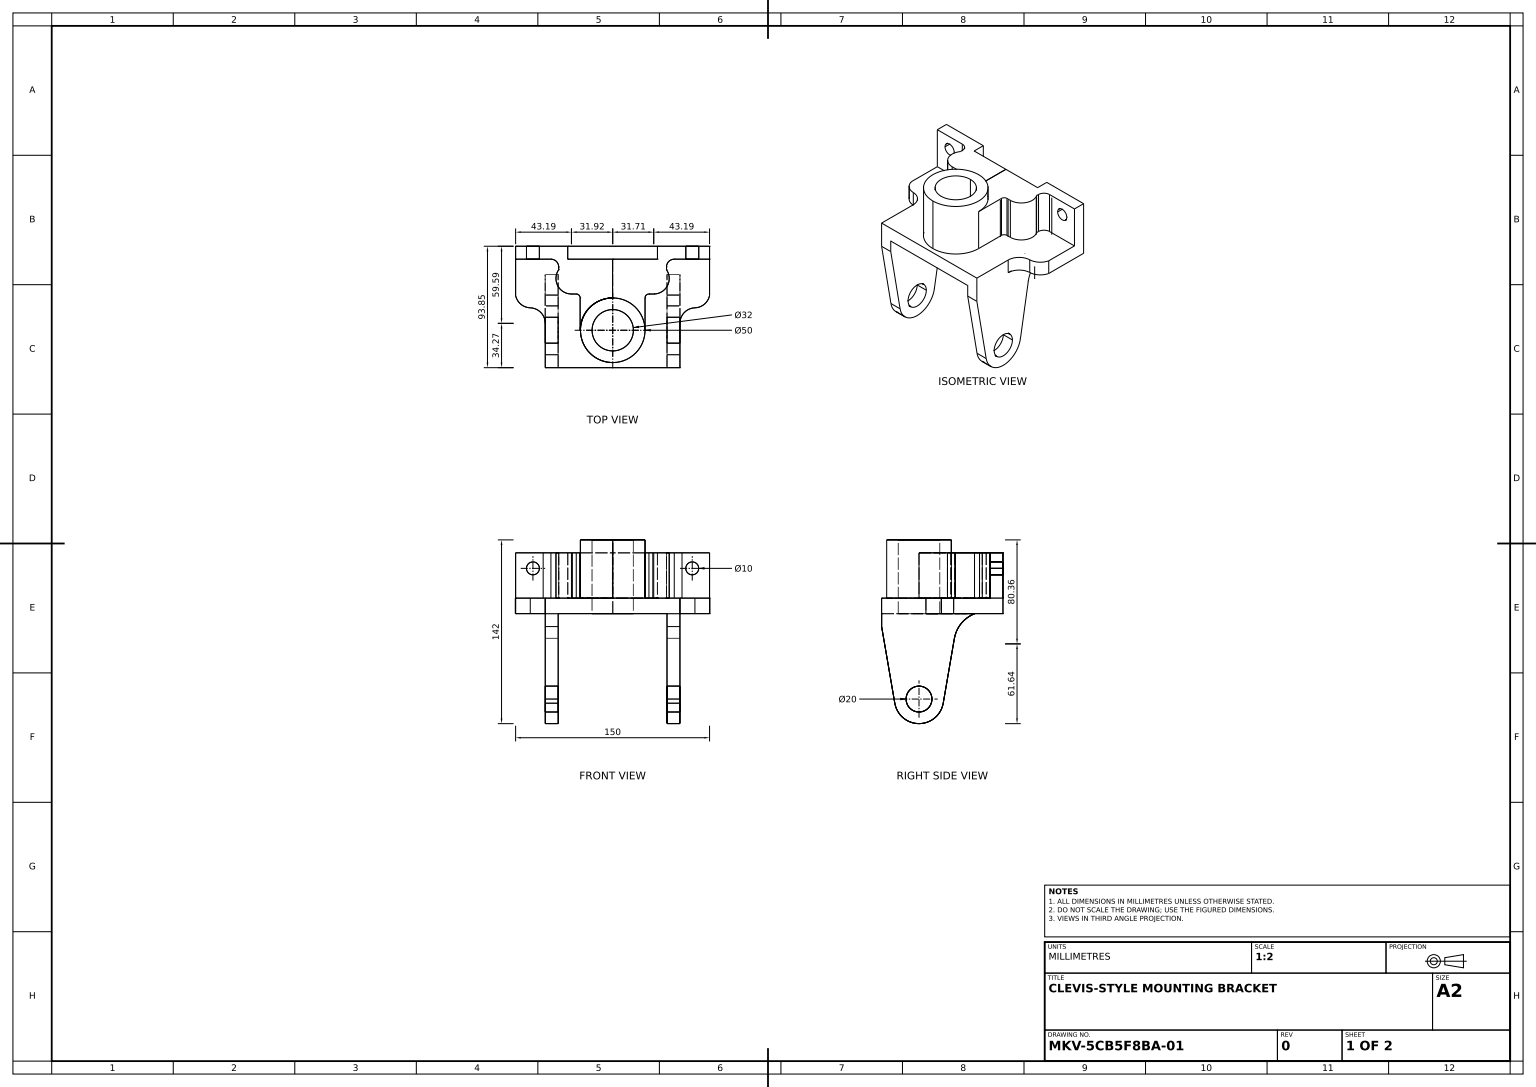
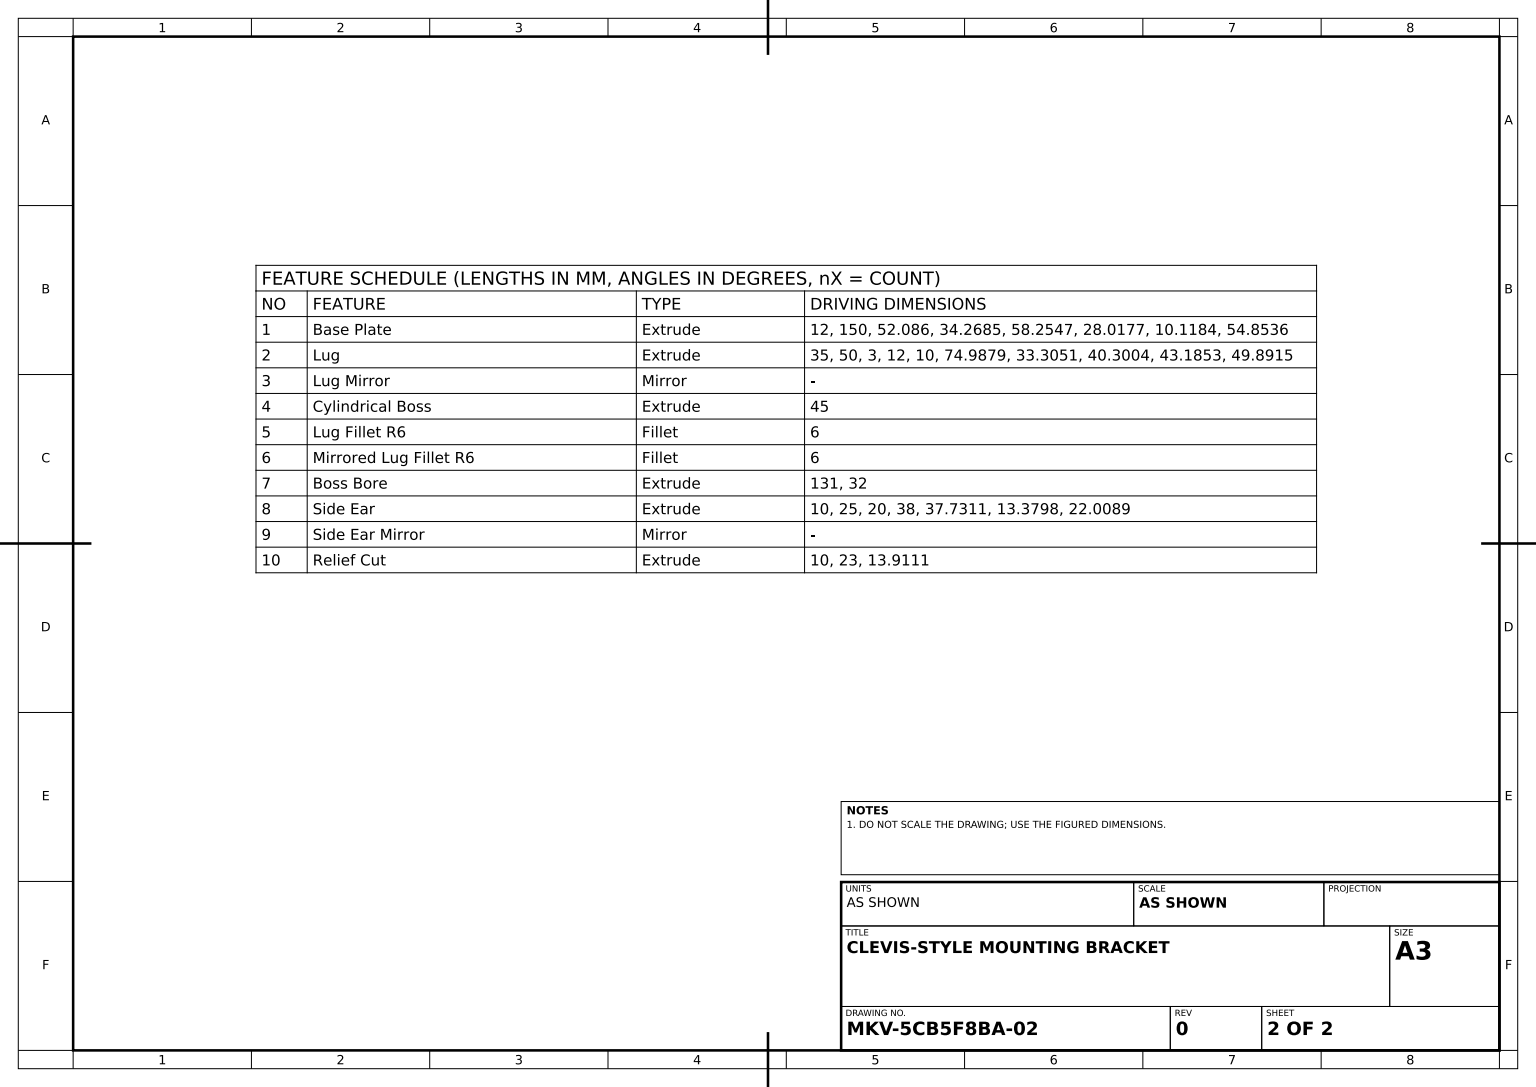
solid
v1 (52.086043,0,-34.268492)
v2 (63.678641,0,-46.261574)
e1 v1 v2 CIRCLE(AX(P(64.086043,0,-34.268492),D(0,-1,0),D(0,0,-1)),12)
v3 (63.678641,12,-46.261574)
e2 v3 v2 LINE
v4 (52.086043,12,-34.268492)
e3 v4 v3 CIRCLE(AX(P(64.086043,12,-34.268492),D(0,-1,0),D(0,0,-1)),12)
e4 v4 v1 LINE
face CYL(AX(P(64.086043,12,-34.268492),D(0,-1,0),D(0,0,-1)),12) rev [e1 -e2 -e3 e4]
v5 (42.086043,-66,-18.923895)
v6 (42.086043,-66,-38.923895)
e5 v5 v6 CIRCLE(AX(P(42.086043,-66,-28.923895),D(1,0,0),D(0,0,-1)),10)
v7 (52.086043,-66,-18.923895)
e6 v5 v7 LINE
v8 (52.086043,-66,-38.923895)
e7 v7 v8 CIRCLE(AX(P(52.086043,-66,-28.923895),D(1,0,0),D(0,0,-1)),10)
e8 v6 v8 LINE
face CYL(AX(P(42.086043,-66,-28.923895),D(1,0,0),D(0,0,-1)),10) rev [-e5 e6 e7 -e8]
v9 (0.108501,0,-12.923895)
v10 (0.108501,0,-44.923895)
e9 v9 v10 CIRCLE(AX(P(0.108501,0,-28.923895),D(0,-1,0),D(0,0,-1)),16)
e10 v10 v9 CIRCLE(AX(P(0.108501,0,-28.923895),D(0,-1,0),D(0,0,-1)),16)
v11 (-42.086043,0,0)
v12 (42.086043,0,0)
e11 v11 v12 LINE
v13 (-42.086043,0,-71.999618)
e12 v11 v13 LINE
v14 (-52.086043,0,-71.999618)
e13 v13 v14 LINE
v15 (-52.086043,0,-34.268492)
e14 v15 v14 LINE
v16 (-63.678641,0,-46.261574)
e15 v16 v15 CIRCLE(AX(P(-64.086043,0,-34.268492),D(0,-1,0),D(0,0,1)),12)
v17 (-75,0,-55.717699)
e16 v17 v16 CIRCLE(AX(P(-63.271238,0,-58.254657),D(0,1,0),D(0,0,-1)),12)
v18 (-75,0,-93.853778)
e17 v18 v17 LINE
v19 (75,0,-93.853778)
e18 v19 v18 LINE
v20 (75,0,-55.717699)
e19 v20 v19 LINE
e20 v2 v20 CIRCLE(AX(P(63.271238,0,-58.254657),D(0,1,0),D(0,0,1)),12)
v21 (52.086043,0,-71.999618)
e21 v1 v21 LINE
v22 (42.086043,0,-71.999618)
e22 v22 v21 LINE
e23 v12 v22 LINE
face PLANE(AX(P(64.086043,0,-34.268492),D(0,-1,0),D(0,0,-1))) [-e9 -e10] [-e11 e12 e13 -e14 -e15 -e16 -e17 -e18 -e19 -e20 -e1 e21 -e22 -e23]
v23 (-42.086043,-66,-38.923895)
v24 (-52.086043,-66,-38.923895)
e24 v23 v24 LINE
v25 (-52.086043,-66,-18.923895)
e25 v25 v24 CIRCLE(AX(P(-52.086043,-66,-28.923895),D(1,0,0),D(0,0,-1)),10)
v26 (-42.086043,-66,-18.923895)
e26 v26 v25 LINE
e27 v26 v23 CIRCLE(AX(P(-42.086043,-66,-28.923895),D(1,0,0),D(0,0,-1)),10)
face CYL(AX(P(-42.086043,-66,-28.923895),D(-1,0,0),D(0,0,1)),10) rev [e24 -e25 -e26 e27]
v27 (47.694924,12,-83.853778)
v28 (75,12,-83.853778)
e28 v27 v28 LINE
v29 (41.694924,12,-77.853778)
e29 v27 v29 CIRCLE(AX(P(47.694924,12,-77.853778),D(0,1,0),D(0,0,-1)),6)
v30 (41.694924,12,-75.734291)
e30 v30 v29 LINE
v31 (31.814716,12,-56.923895)
e31 v31 v30 CIRCLE(AX(P(31.814716,12,-68.923895),D(0,1,0),D(0,0,1)),12)
v32 (28.108501,12,-56.923895)
e32 v32 v31 LINE
v33 (25.108501,12,-53.923895)
e33 v33 v32 CIRCLE(AX(P(28.108501,12,-53.923895),D(0,-1,0),D(0,0,1)),3)
v34 (25.108501,12,-28.923895)
e34 v34 v33 LINE
v35 (0.108501,12,-3.923895)
e35 v35 v34 CIRCLE(AX(P(0.108501,12,-28.923895),D(0,1,0),D(0,0,1)),25)
v36 (0.048176,12,-53.923823)
e36 v36 v35 CIRCLE(AX(P(0.108501,12,-28.923895),D(0,1,0),D(0,0,1)),25)
v37 (0.012065,12,-83.853778)
e37 v37 v36 LINE
v38 (34.69959,12,-83.853778)
e38 v38 v37 LINE
v39 (34.69959,12,-93.853778)
e39 v39 v38 LINE
v40 (-34.69959,12,-93.853778)
e40 v39 v40 LINE
v41 (-34.69959,12,-83.853778)
e41 v40 v41 LINE
v42 (-0.012065,12,-83.853778)
e42 v41 v42 LINE
v43 (-0.048176,12,-53.923823)
e43 v42 v43 LINE
v44 (-0.108501,12,-53.923895)
e44 v44 v43 CIRCLE(AX(P(-0.108501,12,-28.923895),D(0,-1,0),D(0,0,1)),25)
v45 (-25.108501,12,-28.923895)
e45 v45 v44 CIRCLE(AX(P(-0.108501,12,-28.923895),D(0,-1,0),D(0,0,1)),25)
v46 (-25.108501,12,-53.923895)
e46 v45 v46 LINE
v47 (-28.108501,12,-56.923895)
e47 v46 v47 CIRCLE(AX(P(-28.108501,12,-53.923895),D(0,1,0),D(0,0,1)),3)
v48 (-31.814716,12,-56.923895)
e48 v47 v48 LINE
v49 (-41.694924,12,-75.734291)
e49 v48 v49 CIRCLE(AX(P(-31.814716,12,-68.923895),D(0,-1,0),D(0,0,1)),12)
v50 (-41.694924,12,-77.853778)
e50 v49 v50 LINE
v51 (-47.694924,12,-83.853778)
e51 v50 v51 CIRCLE(AX(P(-47.694924,12,-77.853778),D(0,1,0),D(0,0,-1)),6)
v52 (-75,12,-83.853778)
e52 v51 v52 LINE
v53 (-75,12,-55.717699)
e53 v52 v53 LINE
v54 (-63.678641,12,-46.261574)
e54 v53 v54 CIRCLE(AX(P(-63.271238,12,-58.254657),D(0,1,0),D(0,0,-1)),12)
v55 (-52.086043,12,-34.268492)
e55 v54 v55 CIRCLE(AX(P(-64.086043,12,-34.268492),D(0,-1,0),D(0,0,1)),12)
v56 (-52.086043,12,0)
e56 v55 v56 LINE
v57 (52.086043,12,0)
e57 v56 v57 LINE
e58 v57 v4 LINE
v58 (75,12,-55.717699)
e59 v3 v58 CIRCLE(AX(P(63.271238,12,-58.254657),D(0,1,0),D(0,0,1)),12)
e60 v58 v28 LINE
face PLANE(AX(P(64.086043,12,-34.268492),D(0,-1,0),D(0,0,-1))) rev [-e28 e29 -e30 -e31 -e32 -e33 -e34 -e35 -e36 -e37 -e38 -e39 e40 e41 e42 e43 -e44 -e45 e46 e47 e48 e49 e50 e51 e52 e53 e54 e55 e56 e57 e58 e3 e59 e60]
v59 (-0.048176,47,-53.923823)
e61 v59 v43 LINE
v60 (-0.108501,47,-53.923895)
e62 v60 v59 CIRCLE(AX(P(-0.108501,47,-28.923895),D(0,-1,0),D(0,0,1)),25)
e63 v60 v44 LINE
face CYL(AX(P(-0.108501,47,-28.923895),D(0,-1,0),D(0,0,-1)),25) rev [e44 -e61 -e62 e63]
v61 (-28.108501,47,-56.923895)
e64 v61 v47 LINE
v62 (-31.814716,47,-56.923895)
e65 v61 v62 LINE
e66 v62 v48 LINE
face PLANE(AX(P(0,47,-56.923895),D(0,0,1),D(1,0,0))) [-e64 e65 e66 -e48]
v63 (-34.69959,47,-93.853778)
e67 v63 v40 LINE
v64 (-34.69959,47,-83.853778)
e68 v63 v64 LINE
e69 v64 v41 LINE
face PLANE(AX(P(-34.69959,47,0),D(1,0,0),D(0,0,-1))) [-e41 -e67 e68 e69]
v65 (42.086043,-69.224345,-10.199484)
v66 (52.086043,-69.224345,-10.199484)
e70 v65 v66 LINE
v67 (52.086043,-9.993927,0)
e71 v66 v67 LINE
v68 (42.086043,-9.993927,0)
e72 v68 v67 LINE
e73 v65 v68 LINE
face PLANE(AX(P(42.086043,-0.287814,1.671393),D(0,0.16970239,-0.985495357),D(0,0.985495357,0.16970239))) rev [e70 e71 -e72 -e73]
v69 (25.108501,47,-53.923895)
e74 v69 v33 LINE
v70 (25.108501,47,-28.923895)
e75 v70 v69 LINE
e76 v70 v34 LINE
face PLANE(AX(P(25.108501,47,0),D(-1,0,0),D(0,0,1))) rev [-e74 -e75 e76 e34]
e77 v58 v20 LINE
v71 (75,47,-93.853778)
e78 v71 v19 LINE
v72 (75,47,-83.853778)
e79 v72 v71 LINE
e80 v72 v28 LINE
face PLANE(AX(P(75,12,-83.735384),D(-1,0,0),D(0,0,1))) rev [-e60 e77 e19 -e78 -e79 e80]
v73 (42.086043,-19.113828,-56.277343)
e81 v73 v22 CIRCLE(AX(P(42.086043,-23.356388,-80.914727),D(-1,0,0),D(0,0,-1)),25)
v74 (42.086043,-69.224345,-47.648307)
e82 v74 v73 LINE
e83 v65 v74 CIRCLE(AX(P(42.086043,-66,-28.923895),D(1,0,0),D(0,0,-1)),19)
e84 v12 v68 LINE
e85 v6 v5 CIRCLE(AX(P(42.086043,-66,-28.923895),D(1,0,0),D(0,0,-1)),10)
face PLANE(AX(P(42.086043,0,0),D(1,0,0),D(0,0,-1))) rev [e23 -e81 -e82 -e83 e73 -e84] [e85 e5]
v75 (-42.086043,-69.224345,-47.648307)
v76 (-42.086043,-19.113828,-56.277343)
e86 v75 v76 LINE
v77 (-52.086043,-69.224345,-47.648307)
e87 v75 v77 LINE
v78 (-52.086043,-19.113828,-56.277343)
e88 v77 v78 LINE
e89 v76 v78 LINE
face PLANE(AX(P(-42.086043,-9.962332,-57.853231),D(0,0.16970239,0.985495357),D(0,-0.985495357,0.16970239))) rev [-e86 e87 e88 -e89]
face CYL(AX(P(63.271238,12,-58.254657),D(0,-1,0),D(0,0,-1)),12) [-e59 e2 e20 -e77]
v79 (-0.012065,47,-83.853778)
e90 v79 v42 LINE
e91 v79 v59 LINE
face PLANE(AX(P(-0.113235,47,-0.000137),D(0.999999272,0,0.001206505),D(0.001206505,0,-0.999999272))) [-e90 e91 e61 -e43]
v80 (-42.086043,-69.224345,-10.199484)
e92 v80 v75 CIRCLE(AX(P(-42.086043,-66,-28.923895),D(1,0,0),D(0,0,-1)),19)
e93 v76 v13 CIRCLE(AX(P(-42.086043,-23.356388,-80.914727),D(-1,0,0),D(0,0,-1)),25)
v81 (-42.086043,-9.993927,0)
e94 v11 v81 LINE
e95 v80 v81 LINE
e96 v23 v26 CIRCLE(AX(P(-42.086043,-66,-28.923895),D(1,0,0),D(0,0,-1)),10)
face PLANE(AX(P(-42.086043,0,0),D(-1,0,0),D(0,0,-1))) rev [e92 e86 e93 -e12 e94 -e95] [-e96 -e27]
v82 (31.814716,47,-56.923895)
v83 (41.694924,47,-75.734291)
e97 v82 v83 CIRCLE(AX(P(31.814716,47,-68.923895),D(0,1,0),D(0,0,1)),12)
e98 v82 v31 LINE
e99 v83 v30 LINE
face CYL(AX(P(31.814716,47,-68.923895),D(0,-1,0),D(0,0,-1)),12) [-e97 e98 e31 -e99]
v84 (-52.086043,-69.224345,-10.199484)
e100 v80 v84 LINE
e101 v84 v77 CIRCLE(AX(P(-52.086043,-66,-28.923895),D(1,0,0),D(0,0,-1)),19)
face CYL(AX(P(-42.086043,-66,-28.923895),D(-1,0,0),D(0,0,1)),19) [-e87 -e92 e100 e101]
v85 (-41.694924,47,-75.734291)
v86 (-41.694924,47,-77.853778)
e102 v85 v86 LINE
e103 v86 v50 LINE
e104 v85 v49 LINE
face PLANE(AX(P(-41.694924,47,0),D(-1,0,0),D(0,0,1))) [e102 e103 -e50 -e104]
e105 v64 v79 LINE
face PLANE(AX(P(0,47,-83.853778),D(0,0,-1),D(-1,0,0))) [e90 -e42 -e69 e105]
v87 (66.606022,35,-93.853778)
v88 (56.606022,35,-93.853778)
e106 v87 v88 CIRCLE(AX(P(61.606022,35,-93.853778),D(0,0,1),D(1,0,0)),5)
v89 (66.606022,35,-83.853778)
e107 v87 v89 LINE
v90 (56.606022,35,-83.853778)
e108 v89 v90 CIRCLE(AX(P(61.606022,35,-83.853778),D(0,0,1),D(1,0,0)),5)
e109 v88 v90 LINE
face CYL(AX(P(61.606022,35,-93.853778),D(0,0,1),D(1,0,0)),5) rev [-e106 e107 e108 -e109]
v91 (-25.108501,47,-53.923895)
e110 v91 v61 CIRCLE(AX(P(-28.108501,47,-53.923895),D(0,1,0),D(0,0,1)),3)
e111 v91 v46 LINE
face CYL(AX(P(-28.108501,47,-53.923895),D(0,-1,0),D(0,0,-1)),3) rev [e110 e64 -e47 -e111]
v92 (52.086043,-69.224345,-47.648307)
e112 v74 v92 LINE
e113 v66 v92 CIRCLE(AX(P(52.086043,-66,-28.923895),D(1,0,0),D(0,0,-1)),19)
face CYL(AX(P(42.086043,-66,-28.923895),D(1,0,0),D(0,0,-1)),19) [e83 e112 -e113 -e70]
v93 (-56.606022,35,-83.853778)
v94 (-66.606022,35,-83.853778)
e114 v93 v94 CIRCLE(AX(P(-61.606022,35,-83.853778),D(0,0,1),D(-1,0,0)),5)
v95 (-66.606022,35,-93.853778)
e115 v95 v94 LINE
v96 (-56.606022,35,-93.853778)
e116 v96 v95 CIRCLE(AX(P(-61.606022,35,-93.853778),D(0,0,1),D(-1,0,0)),5)
e117 v96 v93 LINE
face CYL(AX(P(-61.606022,35,-93.853778),D(0,0,1),D(1,0,0)),5) rev [e114 -e115 -e116 e117]
e118 v90 v89 CIRCLE(AX(P(61.606022,35,-83.853778),D(0,0,1),D(1,0,0)),5)
v97 (47.694924,47,-83.853778)
e119 v97 v72 LINE
e120 v97 v27 LINE
face PLANE(AX(P(0,47,-83.853778),D(0,0,-1),D(-1,0,0))) rev [-e108 -e118] [-e119 e120 e28 -e80]
e121 v94 v93 CIRCLE(AX(P(-61.606022,35,-83.853778),D(0,0,1),D(-1,0,0)),5)
v98 (-47.694924,47,-83.853778)
e122 v51 v98 LINE
v99 (-75,47,-83.853778)
e123 v98 v99 LINE
e124 v99 v52 LINE
face PLANE(AX(P(0,47,-83.853778),D(0,0,1),D(1,0,0))) [-e121 -e114] [e122 e123 e124 -e52]
v100 (52.086043,-19.113828,-56.277343)
e125 v100 v21 CIRCLE(AX(P(52.086043,-23.356388,-80.914727),D(-1,0,0),D(0,0,-1)),25)
e126 v73 v100 LINE
face CYL(AX(P(42.086043,-23.356388,-80.914727),D(1,0,0),D(0,0,-1)),25) rev [e22 -e125 -e126 e81]
e127 v92 v100 LINE
face PLANE(AX(P(42.086043,-9.962332,-57.853231),D(0,-0.16970239,-0.985495357),D(0,0.985495357,-0.16970239))) [-e127 -e112 e82 e126]
v101 (28.108501,47,-56.923895)
e128 v101 v32 LINE
e129 v101 v82 LINE
face PLANE(AX(P(0,47,-56.923895),D(0,0,-1),D(-1,0,0))) rev [e128 e32 -e98 -e129]
e130 v54 v16 LINE
e131 v55 v15 LINE
face CYL(AX(P(-64.086043,12,-34.268492),D(0,-1,0),D(0,0,-1)),12) rev [e130 e15 -e131 -e55]
e132 v57 v67 LINE
v102 (-52.086043,-9.993927,0)
e133 v56 v102 LINE
e134 v81 v102 LINE
face PLANE(AX(P(0,12,0),D(0,0,-1),D(-1,0,0))) rev [-e132 -e57 e133 -e134 -e94 e11 e84 e72]
v103 (0.108501,57,-3.923895)
v104 (0.108501,57,-53.923895)
e135 v103 v104 CIRCLE(AX(P(0.108501,57,-28.923895),D(0,1,0),D(0,0,1)),25)
e136 v103 v35 LINE
v105 (0.108501,47,-53.923895)
e137 v70 v105 CIRCLE(AX(P(0.108501,47,-28.923895),D(0,1,0),D(0,0,1)),25)
e138 v104 v105 LINE
face CYL(AX(P(0.108501,57,-28.923895),D(0,-1,0),D(0,0,-1)),25) [-e135 e136 e35 -e76 e137 -e138]
v106 (34.69959,47,-83.853778)
v107 (0.012065,47,-83.853778)
e139 v106 v107 LINE
e140 v106 v38 LINE
e141 v107 v37 LINE
face PLANE(AX(P(0,47,-83.853778),D(0,0,1),D(1,0,0))) rev [-e139 e140 e38 -e141]
v108 (0.048176,47,-53.923823)
e142 v105 v108 CIRCLE(AX(P(0.108501,47,-28.923895),D(0,1,0),D(0,0,1)),25)
e143 v108 v36 LINE
e144 v104 v103 CIRCLE(AX(P(0.108501,57,-28.923895),D(0,1,0),D(0,0,1)),25)
face CYL(AX(P(0.108501,57,-28.923895),D(0,-1,0),D(0,0,-1)),25) [e142 e143 e36 -e136 -e144 e138]
e145 v107 v108 LINE
face PLANE(AX(P(0.113235,47,-0.000137),D(0.999999272,0,-0.001206505),D(-0.001206505,0,-0.999999272))) rev [e141 e37 -e143 -e145]
v109 (0.108501,57,-12.923895)
e146 v9 v109 LINE
v110 (0.108501,57,-44.923895)
e147 v109 v110 CIRCLE(AX(P(0.108501,57,-28.923895),D(0,1,0),D(0,0,1)),16)
e148 v10 v110 LINE
face CYL(AX(P(0.108501,-74,-28.923895),D(0,1,0),D(0,0,1)),16) rev [e146 e147 -e148 e10]
e149 v95 v96 CIRCLE(AX(P(-61.606022,35,-93.853778),D(0,0,1),D(-1,0,0)),5)
face CYL(AX(P(-61.606022,35,-93.853778),D(0,0,1),D(1,0,0)),5) rev [e115 e121 -e117 -e149]
e150 v110 v109 CIRCLE(AX(P(0.108501,57,-28.923895),D(0,1,0),D(0,0,1)),16)
face PLANE(AX(P(0.108501,57,-28.923895),D(0,1,0),D(0,0,1))) [-e150 -e147] [e135 e144]
v111 (-25.108501,47,-28.923895)
e151 v111 v60 CIRCLE(AX(P(-0.108501,47,-28.923895),D(0,-1,0),D(0,0,1)),25)
e152 v111 v45 LINE
face CYL(AX(P(-0.108501,47,-28.923895),D(0,-1,0),D(0,0,-1)),25) rev [-e151 e152 e45 -e63]
e153 v111 v91 LINE
face PLANE(AX(P(-25.108501,47,0),D(-1,0,0),D(0,0,1))) [-e152 e153 e111 -e46]
e154 v8 v7 CIRCLE(AX(P(52.086043,-66,-28.923895),D(1,0,0),D(0,0,-1)),10)
face CYL(AX(P(42.086043,-66,-28.923895),D(1,0,0),D(0,0,-1)),10) rev [-e6 -e85 e8 e154]
v112 (41.694924,47,-77.853778)
e155 v29 v112 LINE
e156 v112 v97 CIRCLE(AX(P(47.694924,47,-77.853778),D(0,-1,0),D(0,0,1)),6)
face CYL(AX(P(47.694924,47,-77.853778),D(0,1,0),D(0,0,1)),6) rev [-e155 -e29 -e120 -e156]
e157 v84 v102 LINE
face PLANE(AX(P(-42.086043,-0.287814,1.671393),D(0,-0.16970239,0.985495357),D(0,-0.985495357,-0.16970239))) [-e157 -e100 e95 e134]
e158 v83 v112 LINE
face PLANE(AX(P(41.694924,47,0),D(-1,0,0),D(0,0,1))) rev [e155 -e158 e99 e30]
e159 v53 v17 LINE
face CYL(AX(P(-63.271238,12,-58.254657),D(0,-1,0),D(0,0,-1)),12) [-e54 e159 e16 -e130]
e160 v88 v87 CIRCLE(AX(P(61.606022,35,-93.853778),D(0,0,1),D(1,0,0)),5)
v113 (34.69959,47,-93.853778)
e161 v113 v39 LINE
e162 v71 v113 LINE
v114 (-75,47,-93.853778)
e163 v114 v18 LINE
e164 v114 v63 LINE
face PLANE(AX(P(-75,12,-93.853778),D(0,0,1),D(1,0,0))) rev [e160 e106] [e149 e116] [e67 -e40 -e161 -e162 e78 e18 -e163 e164]
face CYL(AX(P(0.108501,-74,-28.923895),D(0,1,0),D(0,0,1)),16) rev [e148 e150 -e146 e9]
e165 v78 v14 CIRCLE(AX(P(-52.086043,-23.356388,-80.914727),D(-1,0,0),D(0,0,-1)),25)
face CYL(AX(P(-42.086043,-23.356388,-80.914727),D(-1,0,0),D(0,0,1)),25) rev [-e93 e89 e165 -e13]
face CYL(AX(P(61.606022,35,-93.853778),D(0,0,1),D(1,0,0)),5) rev [-e107 -e160 e109 e118]
e166 v99 v114 LINE
face PLANE(AX(P(-75,12,-55.717699),D(1,0,0),D(0,0,-1))) rev [-e159 -e53 -e124 e166 e163 e17]
e167 v98 v86 CIRCLE(AX(P(-47.694924,47,-77.853778),D(0,-1,0),D(0,0,1)),6)
face CYL(AX(P(-47.694924,47,-77.853778),D(0,1,0),D(0,0,1)),6) rev [-e51 -e103 -e167 -e122]
e168 v62 v85 CIRCLE(AX(P(-31.814716,47,-68.923895),D(0,-1,0),D(0,0,1)),12)
face CYL(AX(P(-31.814716,47,-68.923895),D(0,-1,0),D(0,0,-1)),12) [-e66 e168 e104 -e49]
face PLANE(AX(P(52.086043,12,0),D(-1,0,0),D(0,0,1))) rev [e132 -e71 e113 e127 e125 -e21 -e4 -e58] [-e7 -e154]
e169 v24 v25 CIRCLE(AX(P(-52.086043,-66,-28.923895),D(1,0,0),D(0,0,-1)),10)
face CYL(AX(P(-42.086043,-66,-28.923895),D(-1,0,0),D(0,0,1)),10) rev [-e24 e96 e26 -e169]
e170 v69 v101 CIRCLE(AX(P(28.108501,47,-53.923895),D(0,-1,0),D(0,0,1)),3)
face CYL(AX(P(28.108501,47,-53.923895),D(0,-1,0),D(0,0,-1)),3) rev [e33 -e128 -e170 e74]
e171 v113 v106 LINE
face PLANE(AX(P(0,47,0),D(0,1,0),D(0,0,1))) [e170 e129 e97 e158 e156 e119 e79 e162 e171 e139 e145 -e142 -e137 e75]
face PLANE(AX(P(0,47,0),D(0,1,0),D(0,0,1))) [e151 e62 -e91 -e105 -e68 -e164 -e166 -e123 e167 -e102 -e168 -e65 -e110 -e153]
face PLANE(AX(P(-52.086043,12,0),D(1,0,0),D(0,0,-1))) rev [-e165 -e88 -e101 e157 -e133 -e56 e131 e14] [e25 e169]
face PLANE(AX(P(34.69959,47,0),D(1,0,0),D(0,0,-1))) rev [e39 -e140 -e171 e161]
